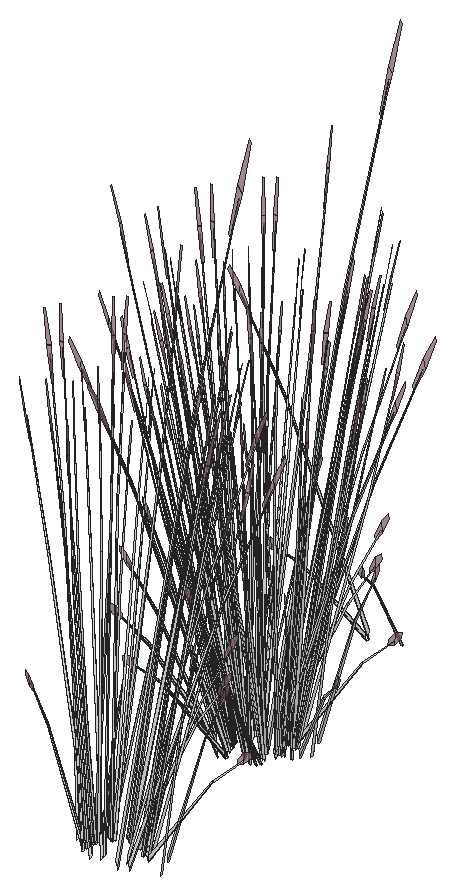
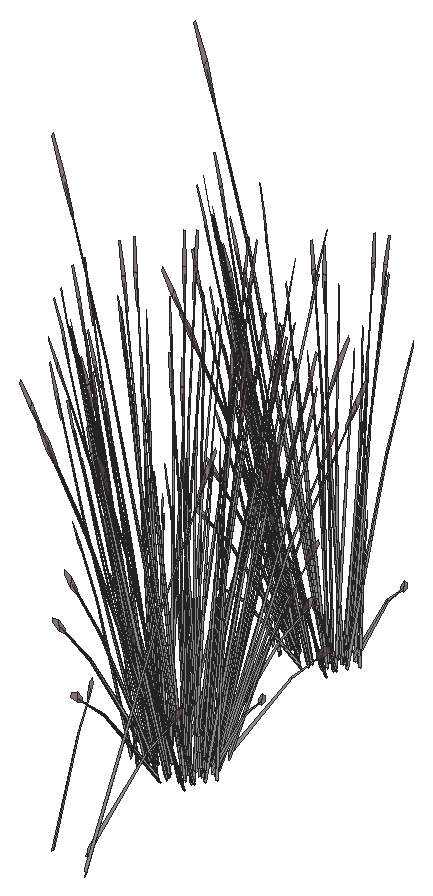
# SketchUp Ruby script. Lengths in inches.
U = 1.inch
M = Sketchup.active_model
def pt(a) = Geom::Point3d.new(a.map { |v| v * U })
def face(e, loops, mat)
  f = e.add_face(loops[0].map { |a| pt(a) })
  loops[1..].each { |l| e.add_face(l.map { |a| pt(a) }).erase! }
  f.material = f.back_material = mat if mat
  f
end
# faces: each face lists its corners as indices into pts; further lists are holes
def faces(e, pts, list, mat = nil) = list.each { |f| face(e, (f[0].is_a?(Array) ? f : [f]).map { |l| l.map { |i| pts[i] } }, mat) }
# xy, xz, yz: faces in a plane at the given z, y or x. An outline is a flat list of corners, or four numbers for a rectangle; further outlines are holes
def ring(l) = l.size == 4 ? [[l[0], l[1]], [l[2], l[1]], [l[2], l[3]], [l[0], l[3]]] : l.each_slice(2).to_a
def flat(e, list, mat, &to3) = list.each { |f| face(e, (f[0].is_a?(Array) ? f : [f]).map { |l| ring(l).map { |u, v| to3.(u, v) } }, mat) }
def xy(e, z, list, mat = nil) = flat(e, list, mat) { |x, y| [x, y, z] }
def xz(e, y, list, mat = nil) = flat(e, list, mat) { |x, z| [x, y, z] }
def yz(e, x, list, mat = nil) = flat(e, list, mat) { |y, z| [x, y, z] }
def lines(e, pts, list) = list.each { |a, b| e.add_line(pt(pts[a]), pt(pts[b])) }
# prism: a flat outline (further loops are holes) pulled along v
def prism(e, loops, v, mat = nil)
  f = face(e, loops, mat); d = Geom::Vector3d.new(v.map { |x| x * U })
  f.pushpull(f.normal.samedirection?(d) ? d.length : -d.length)
end
def box(e, o, s, mat = nil) = prism(e, [[o, [o[0] + s[0], o[1], o[2]], [o[0] + s[0], o[1] + s[1], o[2]], [o[0], o[1] + s[1], o[2]]]], [0, 0, s[2]], mat)
def at(x, y, z, deg = 0) = Geom::Transformation.translation(pt([x, y, z])) * Geom::Transformation.rotation(ORIGIN, Z_AXIS, deg.degrees)
def axes(o, x, y, z) = Geom::Transformation.new([*x, 0, *y, 0, *z, 0, *pt(o).to_a, 1])
def part(name) = M.definitions.add(name)
# library, detail: a bought-in or finely detailed component or shape, given as its bounding box
def library(name, o, s) = part(name).tap { |d| box(d.entities, o, s) }
def detail(e, o, s) = box(e.add_group.entities, o, s)
def put(e, d, t, mat = nil) = e.add_instance(d, t).tap { |i| i.material = mat if mat }
def group(e, t, mat = nil) = e.add_group.tap { |g| g.transformation = t; g.material = mat if mat }.entities
root = M.entities
M.materials.add("LightPink_Translucent").color = [144, 107, 117]
M.materials["LightPink_Translucent"].alpha = 0.75
c1 = part("blade")
p = [[2.15,0.21,22],[0,0.17,0],[0.09,0.45,0],[2.18,0.31,22],[2.29,0.31,22],[0.38,0.45,0],
  [2.48,0.24,33],[2.49,0.24,33],[2.48,0.22,33]]
faces(c1.entities,p,[[0,1,2,3],[4,5,2,3],[6,3,4,7],[8,0,3,6]])
c2 = part("seeds")
p = [[0.3,-0.1,1.38],[-0.01,-0.03,1.59],[-0.01,-0.03,0.03],[0.14,-0.07,-0.07],[0.29,-0.03,3],[0.15,0.01,3.11]]
faces(c2.entities,p,[[0,1,2,3],[1,0,4,5]],"LightPink_Translucent")
c3 = part("blade with seeds")
put(c3.entities,c1,at(0,0,0))
put(c3.entities,c2,axes([2.4,0.25,30.99],[1.5799,-0.05474,1.17369],[-0.12525,1.92788,0.29478],[-0.07173,-0.02425,1.56792]))
put(root,c3,axes([298.46,213.57,151.27],[0.34057,0.13158,0.29918],[-0.09933,0.38387,-0.38624],[-0.13712,0.0352,0.73904]))
put(root,c3,axes([302.71,215.66,150.98],[-0.03706,-0.04129,1.49853],[0.08106,-0.44261,-0.1416],[0.14596,-0.02828,0.26519]))
put(root,c3,axes([297.89,213.86,150.98],[-0.06692,0.06124,1.47793],[0.00569,0.44742,-0.23373],[-0.15339,0.05818,0.11853]))
put(root,c3,axes([298.32,213.4375,151.25],[0.20619,0.42709,-0.10273],[-0.36595,0.20988,-0.57019],[-0.15422,0.05635,0.8664]))
put(root,c3,axes([302.39,215.29,150.32],[-0.07843,-0.39649,-0.0295],[0.37072,-0.09115,-0.13375],[0.07742,0.02514,0.44114]))
put(root,c3,axes([301.43,215.28,151.25],[0.02194,-0.47967,-0.10273],[0.41546,0.01311,-0.57019],[0.16001,0.03332,0.8664]))
put(root,c3,axes([301.36,215.09,151.27],[-0.23317,-0.29531,0.29918],[0.26625,-0.27955,-0.38624],[0.13527,0.04253,0.73904]))
put(root,c3,axes([301.79,214.99,150.98],[0.08791,-0.00798,1.47793],[0.24113,-0.36643,-0.23373],[0.15637,0.04837,0.11853]))
put(root,c3,axes([298.27,214.63,151],[-0.10163,-0.43409,0.40553],[0.39868,-0.07534,0.33437],[-0.1175,0.10209,0.83914]))
put(root,c3,axes([298.19,214.55,151],[-0.28133,-0.19836,0.05432],[0.16379,-0.28248,0.42765],[-0.0902,0.09132,0.65209]))
put(root,c3,axes([298.32,214.02,150.27],[0.14219,-0.09977,1.44779],[0.11971,0.461,0.11706],[-0.22323,0.10419,0.61892]))
put(root,c3,axes([298.52,214.49,151.27],[0.35672,-0.06741,0.29918],[0.09419,0.38534,-0.38624],[-0.10222,0.1035,0.73904]))
put(root,c3,axes([297.14,214.32,150.98],[0.0523,0.01265,1.49853],[0.16179,0.41674,-0.1416],[-0.10706,0.10938,0.26519]))
put(root,c3,axes([301.69,215.24,150.82],[0.23317,0.29531,-0.29918],[-0.26625,0.27955,0.38624],[0.13527,0.04253,0.73904]))
put(root,c3,axes([301.57,215.36,151],[-0.02064,0.35866,0.05432],[-0.3116,-0.00983,0.42765],[0.11936,0.03753,0.65209]))
put(root,c3,axes([298.23,214.71,150.82],[-0.35672,0.06741,-0.29918],[-0.09419,-0.38534,0.38624],[-0.10222,0.1035,0.73904]))
put(root,c3,axes([301.6,215.24,151],[-0.30217,0.31079,0.40553],[-0.2606,-0.33005,0.33437],[0.14177,0.05733,0.83914]))
put(root,c3,axes([300.64,215.6,151.27],[-0.06329,-0.37991,0.29918],[0.36182,-0.10032,-0.38624],[0.09718,0.10887,0.73904]))
put(root,c3,axes([300.86,214.49,150.27],[-0.15222,-0.08126,1.44779],[0.31502,-0.34091,0.11706],[0.19634,0.15379,0.61892]))
put(root,c3,axes([300.88,213.42,150.78],[-0.35411,-0.24507,1.16821],[0.37391,-0.38156,0.50405],[0.11425,0.22994,1.12919]))
put(root,c3,axes([298.33,214.45,151.25],[0.37908,0.26007,-0.10273],[-0.21839,0.37663,-0.57019],[-0.1071,0.13092,0.8664]))
put(root,c3,axes([300.61,215.8,151.25],[0.2442,-0.40372,-0.10273],[0.35364,0.23259,-0.57019],[0.12293,0.11406,0.8664]))
put(root,c3,axes([298.84,214.34,150.27],[0.10236,-0.14492,1.44779],[0.25844,0.39118,0.11706],[-0.17726,0.17814,0.61892]))
put(root,c3,axes([299,215.25,151.27],[0.27728,-0.24833,0.29918],[0.26248,0.28355,-0.38624],[-0.03994,0.14407,0.73904]))
put(root,c3,axes([300.29,216.13,150.98],[0.00121,-0.0571,1.49853],[0.35119,-0.25193,-0.1416],[0.12199,0.08992,0.26519]))
put(root,c3,axes([298.75,215.48,151],[-0.33677,-0.02198,0.05432],[0.00923,-0.33185,0.42765],[-0.03524,0.12712,0.65209]))
put(root,c3,axes([298.85,215.51,151],[-0.29182,-0.32181,0.40553],[0.3099,-0.27755,0.33437],[-0.05383,0.15098,0.83914]))
put(root,c3,axes([299.78,215.66,151.27],[0.12355,-0.36271,0.29918],[0.36044,0.10579,-0.38624],[0.03305,0.14603,0.73904]))
put(root,c3,axes([300.7,215.95,151],[-0.18625,0.29962,0.05432],[-0.26523,-0.17444,0.42765],[0.08575,0.09606,0.65209]))
put(root,c3,axes([300.78,215.86,151],[-0.4076,0.10824,0.40553],[-0.07074,-0.4246,0.33437],[0.09586,0.12514,0.83914]))
put(root,c3,axes([298.77,214.69,150.27],[0.0763,-0.16212,1.44779],[0.3201,0.3355,0.11706],[-0.1444,0.2091,0.61892]))
put(root,c3,axes([299.66,215.99,151],[-0.30197,0.1603,0.05432],[-0.1478,-0.29231,0.42765],[0.02916,0.12885,0.65209]))
put(root,c3,axes([298.85,215.61,150.82],[-0.27728,0.24833,-0.29918],[-0.26248,-0.28355,0.38624],[-0.03994,0.14407,0.73904]))
put(root,c3,axes([297.9,215.53,150.98],[-0.01019,0.09334,1.47793],[0.28908,0.3247,-0.23373],[-0.07568,0.15355,0.11853]))
put(root,c3,axes([298.82,215.32,151.56],[0.45039,0.02337,-0.11403],[-0.01231,0.44247,-0.63292],[-0.03129,0.17041,0.9617]))
put(root,c3,axes([299.66,215.82,151.25],[0.40102,-0.2196,-0.10273],[0.19707,0.38974,-0.57019],[0.05291,0.16424,0.8664]))
put(root,c3,axes([300.23,214.96,150.27],[-0.09368,-0.15143,1.44779],[0.43286,-0.12749,0.11706],[0.09783,0.23774,0.61892]))
put(root,c3,axes([299.82,216.05,150.82],[-0.12355,0.36271,-0.29918],[-0.36044,-0.10579,0.38624],[0.03305,0.14603,0.73904]))
put(root,c3,axes([297.87,216.49,150.98],[0.04649,-0.02848,1.49853],[0.38427,0.18941,-0.1416],[-0.00903,0.15771,0.26519]))
put(root,c3,axes([299.46,215.04,150.27],[-0.01003,-0.18103,1.44779],[0.43473,0.12009,0.11706],[-0.02689,0.25798,0.61892]))
put(root,c3,axes([299.5625,216.6875,150.98],[0.05195,0.07595,1.47793],[0.41921,0.02984,-0.23373],[0.04216,0.1675,0.11853]))
put(root,c3,axes([297.3,227.6,150.27],[0.09368,0.15143,1.44779],[-0.43286,0.12749,0.11706],[-0.09783,-0.23774,0.61892]))
put(root,c3,axes([298.01,226.59,150.98],[-0.06268,-0.06613,1.47793],[-0.4183,0.04193,-0.23373],[-0.06676,-0.15817,0.11853]))
put(root,c3,axes([299.89,227.4,150.98],[-0.00396,-0.09387,1.47793],[-0.33411,-0.2713,-0.23373],[0.05166,-0.16446,0.11853]))
put(root,c3,axes([298.49,227.38,150.82],[0.12355,-0.36271,-0.29918],[0.36044,0.10579,0.38624],[-0.03305,-0.14603,0.73904]))
put(root,c3,axes([298.76,227.86,150.27],[-0.0763,0.16212,1.44779],[-0.3201,-0.3355,0.11706],[0.1444,-0.2091,0.61892]))
put(root,c3,axes([299.8,227.07,150.98],[-0.04162,0.03603,1.49853],[-0.40776,-0.12155,-0.1416],[-0.01476,-0.15722,0.26519]))
put(root,c3,axes([297.58,226.375,150.98],[-0.00765,0.05653,1.49853],[-0.37706,0.20517,-0.1416],[-0.11096,-0.10488,0.26519]))
put(root,c3,axes([298.53,227.47,151],[0.4038,0.12331,0.40553],[-0.13808,0.40538,0.33437],[-0.02427,-0.15942,0.83914]))
put(root,c3,axes([298.65,227.61,151.25],[-0.40102,0.2196,-0.10273],[-0.19707,-0.38974,-0.57019],[-0.05291,-0.16424,0.8664]))
put(root,c3,axes([299.48,228.11,151.25],[-0.45039,-0.02337,-0.10273],[0.01231,-0.44247,-0.57019],[0.03129,-0.17041,0.8664]))
put(root,c3,axes([299.45,227.82,150.82],[0.27728,-0.24833,-0.29918],[0.26248,0.28355,0.38624],[0.03994,-0.14407,0.73904]))
put(root,c3,axes([298.64,227.4375,151],[0.30197,-0.1603,0.05432],[0.1478,0.29231,0.42765],[-0.02916,-0.12885,0.65209]))
put(root,c3,axes([297.45,227.52,150.82],[-0.06329,-0.37991,-0.29918],[0.36182,-0.10032,0.38624],[-0.09718,-0.10887,0.73904]))
put(root,c3,axes([297.61,227.48,151],[0.18625,-0.29962,0.05432],[0.26523,0.17444,0.42765],[-0.08575,-0.09606,0.65209]))
put(root,c3,axes([296.67,228.07,150.27],[0.15222,0.08126,1.44779],[-0.31502,0.34091,0.11706],[-0.19634,-0.15379,0.61892]))
put(root,c3,axes([298.53,227.77,151.27],[-0.12355,0.36271,0.29918],[-0.36044,-0.10579,-0.38624],[-0.03305,-0.14603,0.73904]))
put(root,c3,axes([299.45,227.92,151],[0.29182,0.32181,0.40553],[-0.3099,0.27755,0.33437],[0.05383,-0.15098,0.83914]))
put(root,c3,axes([297.6875,227.45,151.59],[-0.2735,0.45217,-0.11506],[-0.39608,-0.2605,-0.63862],[-0.13768,-0.12775,0.97037]))
put(root,c3,axes([299.56,227.95,151],[0.33677,0.02198,0.05432],[-0.00923,0.33185,0.42765],[0.03524,-0.12712,0.65209]))
put(root,c3,axes([299.31,228.17,151.27],[-0.27728,0.24833,0.29918],[-0.26248,-0.28355,-0.38624],[0.03994,-0.14407,0.73904]))
put(root,c3,axes([296.64,227.32,150.98],[-0.08817,-0.00333,1.47793],[-0.28072,0.33293,-0.23373],[-0.14978,-0.06803,0.11853]))
put(root,c3,axes([299.97,228.98,151.25],[-0.37908,-0.26007,-0.10273],[0.21839,-0.37663,-0.57019],[0.1071,-0.13092,0.8664]))
put(root,c3,axes([297.66,227.83,151.27],[0.06329,0.37991,0.29918],[-0.36182,0.10032,-0.38624],[-0.09718,-0.10887,0.73904]))
put(root,c3,axes([300.91,228.86,150.98],[-0.05353,-0.00358,1.49853],[-0.22227,-0.38383,-0.1416],[0.08926,-0.1262,0.26519]))
put(root,c3,axes([300.08,228.71,150.82],[0.35672,-0.06741,-0.29918],[0.09419,0.38534,0.38624],[0.10222,-0.1035,0.73904]))
put(root,c3,axes([296.73,228.07,151],[0.02064,-0.35866,0.05432],[0.3116,0.00983,0.42765],[-0.11936,-0.03753,0.65209]))
put(root,c3,axes([296.61,228.19,150.82],[-0.23317,-0.29531,-0.29918],[0.26625,-0.27955,0.38624],[-0.13527,-0.04253,0.73904]))
put(root,c3,axes([299.79,228.94,151.27],[-0.35672,0.06741,0.29918],[-0.09419,-0.38534,-0.38624],[0.10222,-0.1035,0.73904]))
put(root,c3,axes([300.11,228.88,151],[0.28133,0.19836,0.05432],[-0.16379,0.28248,0.42765],[0.0902,-0.09132,0.65209]))
put(root,c3,axes([300.03,228.8,151],[0.10163,0.43409,0.40553],[-0.39868,0.07534,0.33437],[0.1175,-0.10209,0.83914]))
put(root,c3,axes([301.11,229.32,150.98],[0.05687,-0.07184,1.47793],[-0.07279,-0.44069,-0.23373],[0.14268,-0.08356,0.11853]))
put(root,c3,axes([296.3,227.6,150.98],[0.03038,0.04707,1.49853],[-0.14646,0.42312,-0.1416],[-0.14833,0.00306,0.26519]))
put(root,c3,axes([296.94,228.34,151.27],[0.23317,0.29531,0.29918],[-0.26625,0.27955,-0.38624],[-0.13527,-0.04253,0.73904]))
put(root,c3,axes([296.88,228.15,151.25],[-0.02194,0.47967,-0.10273],[-0.41546,-0.01311,-0.57019],[-0.16001,-0.03332,0.8664]))
put(root,c3,axes([299.99,229.99,151.25],[-0.20619,-0.42709,-0.10273],[0.36595,-0.20988,-0.57019],[0.15422,-0.05635,0.8664]))
put(root,c3,axes([296.35,228.8125,150.27],[0.16998,-0.01068,1.44779],[-0.11276,0.46299,0.11706],[-0.24224,-0.02864,0.61892]))
put(root,c3,axes([299.84,229.86,151.27],[-0.34057,-0.13158,0.29918],[0.09933,-0.38387,-0.38624],[0.13712,-0.0352,0.73904]))
put(root,c3,axes([296.28,229.16,151],[0.11578,-0.43006,0.40553],[0.38064,0.14706,0.33437],[-0.14969,0.02584,0.83914]))
put(root,c3,axes([296.25,229.05,151],[-0.15051,-0.3216,0.05432],[0.27447,-0.15741,0.42765],[-0.12099,0.03106,0.65209]))
put(root,c3,axes([300.2,229.82,150.82],[0.34057,0.13158,-0.29918],[-0.09933,0.38387,0.38624],[0.13712,-0.0352,0.73904]))
put(root,c3,axes([296.2,229.21,150.82],[-0.34057,-0.13158,-0.29918],[0.09933,-0.38387,0.38624],[-0.13712,0.0352,0.73904]))
put(root,c3,axes([299.27,229.35,150.27],[-0.16998,0.01068,1.44779],[0.11276,-0.46299,0.11706],[0.24224,0.02864,0.61892]))
put(root,c3,axes([300.15,229.98,151],[0.15051,0.3216,0.05432],[-0.27447,0.15741,0.42765],[0.12099,-0.03106,0.65209]))
put(root,c3,axes([300.125,229.87,151],[-0.11578,0.43006,0.40553],[-0.38064,-0.14706,0.33437],[0.14969,-0.02584,0.83914]))
put(root,c3,axes([296.56,229.17,151.27],[0.34057,0.13158,0.29918],[-0.09933,0.38387,-0.38624],[-0.13712,0.0352,0.73904]))
put(root,c3,axes([300.81,231.26,150.98],[-0.03706,-0.04129,1.49853],[0.08106,-0.44261,-0.1416],[0.14596,-0.02828,0.26519]))
put(root,c3,axes([295.98,229.47,150.98],[-0.06692,0.06124,1.47793],[0.00569,0.44742,-0.23373],[-0.15339,0.05818,0.11853]))
put(root,c3,axes([296.41,229.04,151.25],[0.20619,0.42709,-0.10273],[-0.36595,0.20988,-0.57019],[-0.15422,0.05635,0.8664]))
put(root,c3,axes([300.49,230.89,150.32],[-0.07843,-0.39649,-0.0295],[0.37072,-0.09115,-0.13375],[0.07742,0.02514,0.44114]))
put(root,c3,axes([299.52,230.88,151.25],[0.02194,-0.47967,-0.10273],[0.41546,0.01311,-0.57019],[0.16001,0.03332,0.8664]))
put(root,c3,axes([299.46,230.69,151.27],[-0.23317,-0.29531,0.29918],[0.26625,-0.27955,-0.38624],[0.13527,0.04253,0.73904]))
put(root,c3,axes([299.89,230.59,150.98],[0.08791,-0.00798,1.47793],[0.24113,-0.36643,-0.23373],[0.15637,0.04837,0.11853]))
put(root,c3,axes([296.37,230.23,151],[-0.10163,-0.43409,0.40553],[0.39868,-0.07534,0.33437],[-0.1175,0.10209,0.83914]))
put(root,c3,axes([296.29,230.15,151],[-0.28133,-0.19836,0.05432],[0.16379,-0.28248,0.42765],[-0.0902,0.09132,0.65209]))
put(root,c3,axes([296.42,229.63,150.27],[0.14219,-0.09977,1.44779],[0.11971,0.461,0.11706],[-0.22323,0.10419,0.61892]))
put(root,c3,axes([296.62,230.09,151.27],[0.35672,-0.06741,0.29918],[0.09419,0.38534,-0.38624],[-0.10222,0.1035,0.73904]))
put(root,c3,axes([295.24,229.92,150.98],[0.0523,0.01265,1.49853],[0.16179,0.41674,-0.1416],[-0.10706,0.10938,0.26519]))
put(root,c3,axes([299.79,230.85,150.82],[0.23317,0.29531,-0.29918],[-0.26625,0.27955,0.38624],[0.13527,0.04253,0.73904]))
put(root,c3,axes([299.67,230.96,151],[-0.02064,0.35866,0.05432],[-0.3116,-0.00983,0.42765],[0.11936,0.03753,0.65209]))
put(root,c3,axes([296.32,230.32,150.82],[-0.35672,0.06741,-0.29918],[-0.09419,-0.38534,0.38624],[-0.10222,0.1035,0.73904]))
put(root,c3,axes([299.7,230.85,151],[-0.30217,0.31079,0.40553],[-0.2606,-0.33005,0.33437],[0.14177,0.05733,0.83914]))
put(root,c3,axes([298.74,231.2,151.27],[-0.06329,-0.37991,0.29918],[0.36182,-0.10032,-0.38624],[0.09718,0.10887,0.73904]))
put(root,c3,axes([298.95,230.09,150.27],[-0.15222,-0.08126,1.44779],[0.31502,-0.34091,0.11706],[0.19634,0.15379,0.61892]))
put(root,c3,axes([298.98,229.02,150.78],[-0.35411,-0.24507,1.16821],[0.37391,-0.38156,0.50405],[0.11425,0.22994,1.12919]))
put(root,c3,axes([296.43,230.05,151.25],[0.37908,0.26007,-0.10273],[-0.21839,0.37663,-0.57019],[-0.1071,0.13092,0.8664]))
put(root,c3,axes([298.71,231.4,151.25],[0.2442,-0.40372,-0.10273],[0.35364,0.23259,-0.57019],[0.12293,0.11406,0.8664]))
put(root,c3,axes([296.94,229.9375,150.27],[0.10236,-0.14492,1.44779],[0.25844,0.39118,0.11706],[-0.17726,0.17814,0.61892]))
put(root,c3,axes([297.1,230.86,151.27],[0.27728,-0.24833,0.29918],[0.26248,0.28355,-0.38624],[-0.03994,0.14407,0.73904]))
put(root,c3,axes([298.39,231.74,150.98],[0.00121,-0.0571,1.49853],[0.35119,-0.25193,-0.1416],[0.12199,0.08992,0.26519]))
put(root,c3,axes([296.85,231.08,151],[-0.33677,-0.02198,0.05432],[0.00923,-0.33185,0.42765],[-0.03524,0.12712,0.65209]))
put(root,c3,axes([296.95,231.11,151],[-0.29182,-0.32181,0.40553],[0.3099,-0.27755,0.33437],[-0.05383,0.15098,0.83914]))
put(root,c3,axes([297.875,231.27,151.27],[0.12355,-0.36271,0.29918],[0.36044,0.10579,-0.38624],[0.03305,0.14603,0.73904]))
put(root,c3,axes([298.8,231.55,151],[-0.18625,0.29962,0.05432],[-0.26523,-0.17444,0.42765],[0.08575,0.09606,0.65209]))
put(root,c3,axes([298.875,231.47,151],[-0.4076,0.10824,0.40553],[-0.07074,-0.4246,0.33437],[0.09586,0.12514,0.83914]))
put(root,c3,axes([296.86,230.29,150.27],[0.0763,-0.16212,1.44779],[0.3201,0.3355,0.11706],[-0.1444,0.2091,0.61892]))
put(root,c3,axes([297.76,231.59,151],[-0.30197,0.1603,0.05432],[-0.1478,-0.29231,0.42765],[0.02916,0.12885,0.65209]))
put(root,c3,axes([296.95,231.21,150.82],[-0.27728,0.24833,-0.29918],[-0.26248,-0.28355,0.38624],[-0.03994,0.14407,0.73904]))
put(root,c3,axes([296,231.14,150.98],[-0.01019,0.09334,1.47793],[0.28908,0.3247,-0.23373],[-0.07568,0.15355,0.11853]))
put(root,c3,axes([296.92,230.92,151.56],[0.45039,0.02337,-0.11403],[-0.01231,0.44247,-0.63292],[-0.03129,0.17041,0.9617]))
put(root,c3,axes([297.75,231.42,151.25],[0.40102,-0.2196,-0.10273],[0.19707,0.38974,-0.57019],[0.05291,0.16424,0.8664]))
put(root,c3,axes([298.33,230.5625,150.27],[-0.09368,-0.15143,1.44779],[0.43286,-0.12749,0.11706],[0.09783,0.23774,0.61892]))
put(root,c3,axes([297.91,231.65,150.82],[-0.12355,0.36271,-0.29918],[-0.36044,-0.10579,0.38624],[0.03305,0.14603,0.73904]))
put(root,c3,axes([295.96,232.09,150.98],[0.04649,-0.02848,1.49853],[0.38427,0.18941,-0.1416],[-0.00903,0.15771,0.26519]))
put(root,c3,axes([297.5625,230.64,150.27],[-0.01003,-0.18103,1.44779],[0.43473,0.12009,0.11706],[-0.02689,0.25798,0.61892]))
put(root,c3,axes([297.66,232.29,150.98],[0.05195,0.07595,1.47793],[0.41921,0.02984,-0.23373],[0.04216,0.1675,0.11853]))
put(root,c3,axes([295.07,242.76,150.27],[0.09368,0.15143,1.44779],[-0.43286,0.12749,0.11706],[-0.09783,-0.23774,0.61892]))
put(root,c3,axes([295.78,241.75,150.98],[-0.06268,-0.06613,1.47793],[-0.4183,0.04193,-0.23373],[-0.06676,-0.15817,0.11853]))
put(root,c3,axes([297.66,242.57,150.98],[-0.00396,-0.09387,1.47793],[-0.33411,-0.2713,-0.23373],[0.05166,-0.16446,0.11853]))
